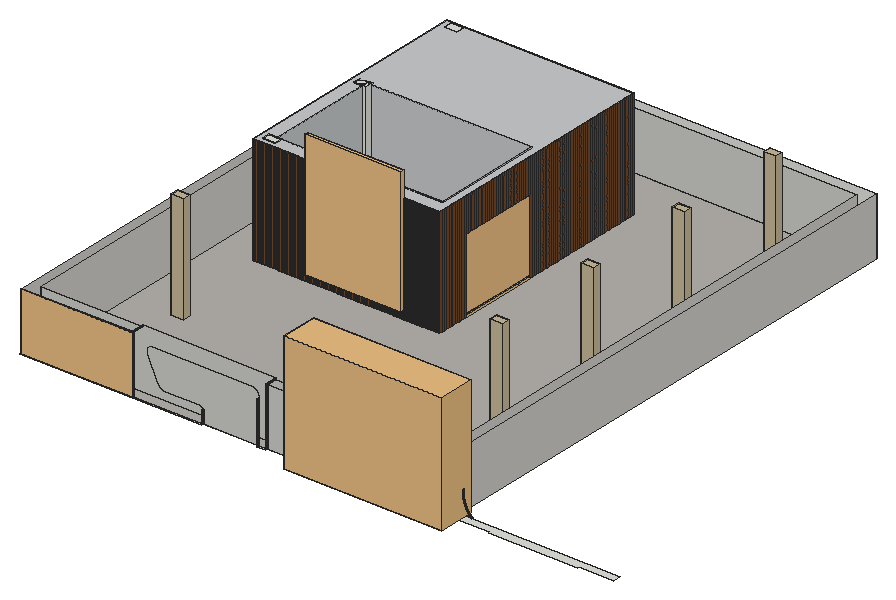
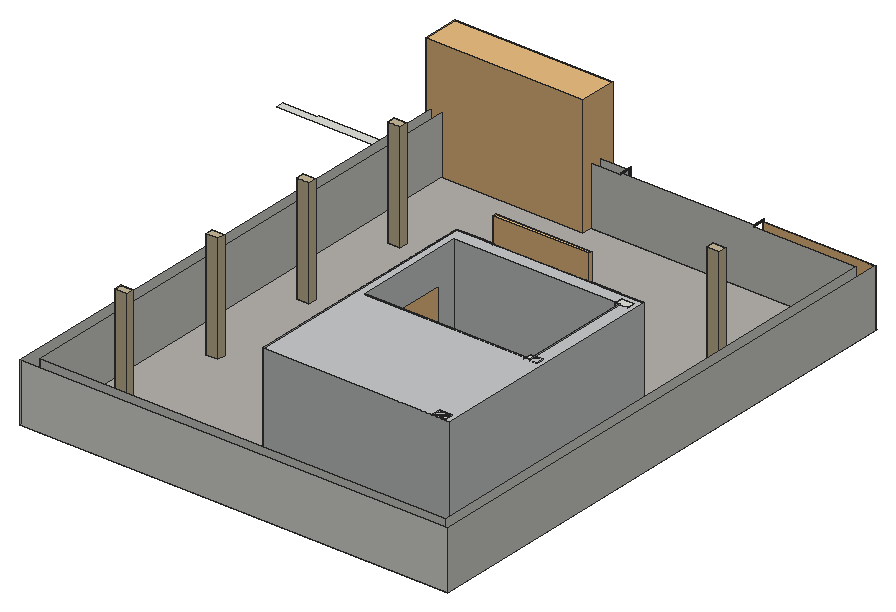
# SketchUp Ruby script. Lengths in inches.
U = 1.inch
M = Sketchup.active_model
def pt(a) = Geom::Point3d.new(a.map { |v| v * U })
def face(e, loops, mat)
  f = e.add_face(loops[0].map { |a| pt(a) })
  loops[1..].each { |l| e.add_face(l.map { |a| pt(a) }).erase! }
  f.material = f.back_material = mat if mat
  f
end
# faces: each face lists its corners as indices into pts; further lists are holes
def faces(e, pts, list, mat = nil) = list.each { |f| face(e, (f[0].is_a?(Array) ? f : [f]).map { |l| l.map { |i| pts[i] } }, mat) }
# xy, xz, yz: faces in a plane at the given z, y or x. An outline is a flat list of corners, or four numbers for a rectangle; further outlines are holes
def ring(l) = l.size == 4 ? [[l[0], l[1]], [l[2], l[1]], [l[2], l[3]], [l[0], l[3]]] : l.each_slice(2).to_a
def flat(e, list, mat, &to3) = list.each { |f| face(e, (f[0].is_a?(Array) ? f : [f]).map { |l| ring(l).map { |u, v| to3.(u, v) } }, mat) }
def xy(e, z, list, mat = nil) = flat(e, list, mat) { |x, y| [x, y, z] }
def xz(e, y, list, mat = nil) = flat(e, list, mat) { |x, z| [x, y, z] }
def yz(e, x, list, mat = nil) = flat(e, list, mat) { |y, z| [x, y, z] }
def lines(e, pts, list) = list.each { |a, b| e.add_line(pt(pts[a]), pt(pts[b])) }
# prism: a flat outline (further loops are holes) pulled along v
def prism(e, loops, v, mat = nil)
  f = face(e, loops, mat); d = Geom::Vector3d.new(v.map { |x| x * U })
  f.pushpull(f.normal.samedirection?(d) ? d.length : -d.length)
end
def box(e, o, s, mat = nil) = prism(e, [[o, [o[0] + s[0], o[1], o[2]], [o[0] + s[0], o[1] + s[1], o[2]], [o[0], o[1] + s[1], o[2]]]], [0, 0, s[2]], mat)
def at(x, y, z, deg = 0) = Geom::Transformation.translation(pt([x, y, z])) * Geom::Transformation.rotation(ORIGIN, Z_AXIS, deg.degrees)
def axes(o, x, y, z) = Geom::Transformation.new([*x, 0, *y, 0, *z, 0, *pt(o).to_a, 1])
def part(name) = M.definitions.add(name)
# library, detail: a bought-in or finely detailed component or shape, given as its bounding box
def library(name, o, s) = part(name).tap { |d| box(d.entities, o, s) }
def detail(e, o, s) = box(e.add_group.entities, o, s)
def put(e, d, t, mat = nil) = e.add_instance(d, t).tap { |i| i.material = mat if mat }
def group(e, t, mat = nil) = e.add_group.tap { |g| g.transformation = t; g.material = mat if mat }.entities
root = M.entities
M.materials.add("1443 AP 8258 WINTER MOON").color = [199, 202, 203]
M.materials.add("[Granite Dark Gray]").color = [51, 50, 50]
M.materials.add("[Quartz Light Brown]").color = [199, 184, 152]
M.materials.add("[Stone Sandstone Ashlar Light]").color = [206, 205, 201]
M.materials.add("[Tile Travertine 2 inch]").color = [181, 178, 172]
M.materials.add("[Wood Cherry Original]").color = [118, 74, 44]
c1 = library("Group\#32",[0,-1,0],[125.5,1,65])
c2 = library("cong+trinh+1",[39.36,9.05,6.78],[177.14,41.14,133.75])
c3 = part("5")
box(c3.entities,[0,0,0],[14,9,121.75])
c4 = library("Plant wall",[-73.82,-5.93,-13.13],[107,4.1,140.96])
c5 = part("Group519\#1")
box(c5.entities,[-105,-60.875,0],[2.5,121.75,0.5])
c6 = part("Group520\#1")
box(c6.entities,[-102,-60.875,0],[2.5,121.75,0.5])
c7 = part("Group521\#1")
box(c7.entities,[-99,-60.875,0],[2.5,121.75,0.5])
c8 = part("Group522\#1")
box(c8.entities,[-96,-60.875,0],[2.5,121.75,0.5])
c9 = part("Group523\#1")
box(c9.entities,[-93,-60.875,0],[2.5,121.75,0.5])
c10 = part("Group524\#1")
box(c10.entities,[-90,-60.875,0],[2.5,121.75,0.5])
c11 = part("Group525\#1")
box(c11.entities,[-87,-60.875,0],[2.5,121.75,0.5])
c12 = part("Group526\#1")
box(c12.entities,[-84,-60.875,0],[2.5,121.75,0.5])
c13 = part("Group527\#1")
box(c13.entities,[-81,-60.875,0],[2.5,121.75,0.5])
c14 = part("Group528\#1")
box(c14.entities,[-78,-60.875,0],[2.5,121.75,0.5])
c15 = part("Group529\#1")
box(c15.entities,[-75,-60.875,0],[2.5,121.75,0.5])
c16 = part("Group530\#1")
box(c16.entities,[-72,-60.875,0],[2.5,121.75,0.5])
c17 = part("Group531\#1")
box(c17.entities,[-69,-60.875,0],[2.5,121.75,0.5])
c18 = part("Group532\#1")
box(c18.entities,[-66,-60.875,0],[2.5,121.75,0.5])
c19 = part("Group533\#1")
box(c19.entities,[-63,-60.875,0],[2.5,121.75,0.5])
c20 = part("Group534\#1")
box(c20.entities,[-60,-60.875,0],[2.5,121.75,0.5])
c21 = part("Group535\#1")
box(c21.entities,[-57,-60.875,0],[2.5,121.75,0.5])
c22 = part("Group536\#1")
box(c22.entities,[-54,-60.875,0],[2.5,121.75,0.5])
c23 = part("Group537\#1")
box(c23.entities,[-51,-60.875,0],[2.5,121.75,0.5])
c24 = part("Group538\#1")
box(c24.entities,[-48,-60.875,0],[2.5,121.75,0.5])
c25 = part("Group539\#1")
box(c25.entities,[-45,-60.875,0],[2.5,121.75,0.5])
c26 = part("Group540\#1")
box(c26.entities,[-42,-60.875,0],[2.5,121.75,0.5])
c27 = part("Group541\#1")
xy(c27.entities,0,[[-39,-60.875,-36.5,-36.875]])
xy(c27.entities,0.5,[[-39,-60.875,-36.5,-36.875]])
xz(c27.entities,-60.875,[[-39,0,-36.5,0.5]])
yz(c27.entities,-39,[[-60.875,0,-36.875,0.5],[-36.875,0,60.875,0.5]])
yz(c27.entities,-36.5,[[-60.875,0,-36.875,0.5]])
c28 = part("Group542\#1")
box(c28.entities,[-36,-60.875,0],[2.5,24,0.5])
c29 = part("Group543\#1")
box(c29.entities,[-33,-60.875,0],[2.5,24,0.5])
c30 = part("Group544\#1")
box(c30.entities,[-30,-60.875,0],[2.5,24,0.5])
c31 = part("Group545\#1")
box(c31.entities,[-27,-60.875,0],[2.5,24,0.5])
c32 = part("Group546\#1")
box(c32.entities,[-24,-60.875,0],[2.5,24,0.5])
c33 = part("Group547\#1")
box(c33.entities,[-21,-60.875,0],[2.5,24,0.5])
c34 = part("Group548\#1")
box(c34.entities,[-18,-60.875,0],[2.5,24,0.5])
c35 = part("Group549\#1")
box(c35.entities,[-15,-60.875,0],[2.5,24,0.5])
c36 = part("Group550\#1")
box(c36.entities,[-12,-60.875,0],[2.5,24,0.5])
c37 = part("Group551\#1")
box(c37.entities,[-9,-60.875,0],[2.5,24,0.5])
c38 = part("Group552\#1")
box(c38.entities,[-6,-60.875,0],[2.5,24,0.5])
c39 = part("Group553\#1")
box(c39.entities,[-3,-60.875,0],[2.5,24,0.5])
c40 = part("Group554\#1")
box(c40.entities,[0,-60.875,0],[2.5,24,0.5])
c41 = part("Group555\#1")
box(c41.entities,[3,-60.875,0],[2.5,24,0.5])
c42 = part("Group556\#1")
box(c42.entities,[6,-60.875,0],[2.5,24,0.5])
c43 = part("Group557\#1")
box(c43.entities,[9,-60.875,0],[2.5,24,0.5])
c44 = part("Group558\#1")
box(c44.entities,[12,-60.875,0],[2.5,24,0.5])
c45 = part("Group559\#1")
box(c45.entities,[15,-60.875,0],[2.5,24,0.5])
c46 = part("Group560\#1")
box(c46.entities,[18,-60.875,0],[2.5,24,0.5])
c47 = part("Group561\#1")
box(c47.entities,[21,-60.875,0],[2.5,24,0.5])
c48 = part("Group562\#1")
box(c48.entities,[24,-60.875,0],[2.5,24,0.5])
c49 = part("Group563\#1")
box(c49.entities,[27,-60.875,0],[2.5,24,0.5])
c50 = part("Group564\#1")
box(c50.entities,[30,-60.875,0],[2.5,24,0.5])
c51 = part("Group565\#1")
box(c51.entities,[33,-60.875,0],[2.5,24,0.5])
c52 = part("Group566\#1")
box(c52.entities,[36,-60.875,0],[2.5,24,0.5])
c53 = part("Group567\#1")
box(c53.entities,[39,-60.875,0],[2.5,24,0.5])
c54 = part("Group568\#1")
box(c54.entities,[42,-60.875,0],[2.5,24,0.5])
c55 = part("Group569\#1")
box(c55.entities,[45,-60.875,0],[2.5,24,0.5])
c56 = part("Group570\#1")
box(c56.entities,[48,-60.875,0],[2.5,24,0.5])
c57 = part("Group571\#1")
box(c57.entities,[51,-60.875,0],[2.5,24,0.5])
c58 = part("Group572\#1")
box(c58.entities,[54,-60.875,0],[2.5,24,0.5])
c59 = part("Group573\#1")
prism(c59.entities,[[[57,-36.875,0],[57,60.875,0],[59.5,60.875,0],[59.5,-60.875,0],[57,-60.875,0]]],[0,0,0.5])
c60 = part("Group574\#1")
box(c60.entities,[60,-60.875,0],[2.5,121.75,0.5])
c61 = part("Group575\#1")
box(c61.entities,[63,-60.875,0],[2.5,121.75,0.5])
c62 = part("Group576\#1")
box(c62.entities,[66,-60.875,0],[2.5,121.75,0.5])
c63 = part("Group577\#1")
box(c63.entities,[69,-60.875,0],[2.5,121.75,0.5])
c64 = part("Group578\#1")
box(c64.entities,[72,-60.875,0],[2.5,121.75,0.5])
c65 = part("Group579\#1")
box(c65.entities,[75,-60.875,0],[2.5,121.75,0.5])
c66 = part("Group580\#1")
box(c66.entities,[78,-60.875,0],[2.5,121.75,0.5])
c67 = part("Group581\#1")
box(c67.entities,[81,-60.875,0],[2.5,121.75,0.5])
c68 = part("Group582\#1")
box(c68.entities,[84,-60.875,0],[2.5,121.75,0.5])
c69 = part("Group583\#1")
box(c69.entities,[87,-60.875,0],[2.5,121.75,0.5])
c70 = part("Group584\#1")
box(c70.entities,[90,-60.875,0],[2.5,121.75,0.5])
c71 = part("Group585\#1")
box(c71.entities,[93,-60.875,0],[2.5,121.75,0.5])
c72 = part("Group586\#1")
box(c72.entities,[96,-60.875,0],[2.5,121.75,0.5])
c73 = part("Group587\#1")
box(c73.entities,[99,-60.875,0],[2.5,121.75,0.5])
c74 = part("Group588\#1")
box(c74.entities,[102,-60.875,0],[2.5,121.75,0.5])
c75 = part("Group517\#1")
put(c75.entities,c5,at(0,0,0))
put(c75.entities,c6,at(0,0,0))
put(c75.entities,c7,at(0,0,0))
put(c75.entities,c8,at(0,0,0))
put(c75.entities,c9,at(0,0,0))
put(c75.entities,c10,at(0,0,0))
put(c75.entities,c11,at(0,0,0))
put(c75.entities,c12,at(0,0,0))
put(c75.entities,c13,at(0,0,0))
put(c75.entities,c14,at(0,0,0))
put(c75.entities,c15,at(0,0,0))
put(c75.entities,c16,at(0,0,0))
put(c75.entities,c17,at(0,0,0))
put(c75.entities,c18,at(0,0,0))
put(c75.entities,c19,at(0,0,0))
put(c75.entities,c20,at(0,0,0))
put(c75.entities,c21,at(0,0,0))
put(c75.entities,c22,at(0,0,0))
put(c75.entities,c23,at(0,0,0))
put(c75.entities,c24,at(0,0,0))
put(c75.entities,c25,at(0,0,0))
put(c75.entities,c26,at(0,0,0))
put(c75.entities,c27,at(0,0,0))
put(c75.entities,c28,at(0,0,0))
put(c75.entities,c29,at(0,0,0))
put(c75.entities,c30,at(0,0,0))
put(c75.entities,c31,at(0,0,0))
put(c75.entities,c32,at(0,0,0))
put(c75.entities,c33,at(0,0,0))
put(c75.entities,c34,at(0,0,0))
put(c75.entities,c35,at(0,0,0))
put(c75.entities,c36,at(0,0,0))
put(c75.entities,c37,at(0,0,0))
put(c75.entities,c38,at(0,0,0))
put(c75.entities,c39,at(0,0,0))
put(c75.entities,c40,at(0,0,0))
put(c75.entities,c41,at(0,0,0))
put(c75.entities,c42,at(0,0,0))
put(c75.entities,c43,at(0,0,0))
put(c75.entities,c44,at(0,0,0))
put(c75.entities,c45,at(0,0,0))
put(c75.entities,c46,at(0,0,0))
put(c75.entities,c47,at(0,0,0))
put(c75.entities,c48,at(0,0,0))
put(c75.entities,c49,at(0,0,0))
put(c75.entities,c50,at(0,0,0))
put(c75.entities,c51,at(0,0,0))
put(c75.entities,c52,at(0,0,0))
put(c75.entities,c53,at(0,0,0))
put(c75.entities,c54,at(0,0,0))
put(c75.entities,c55,at(0,0,0))
put(c75.entities,c56,at(0,0,0))
put(c75.entities,c57,at(0,0,0))
put(c75.entities,c58,at(0,0,0))
put(c75.entities,c59,at(0,0,0))
put(c75.entities,c60,at(0,0,0))
put(c75.entities,c61,at(0,0,0))
put(c75.entities,c62,at(0,0,0))
put(c75.entities,c63,at(0,0,0))
put(c75.entities,c64,at(0,0,0))
put(c75.entities,c65,at(0,0,0))
put(c75.entities,c66,at(0,0,0))
put(c75.entities,c67,at(0,0,0))
put(c75.entities,c68,at(0,0,0))
put(c75.entities,c69,at(0,0,0))
put(c75.entities,c70,at(0,0,0))
put(c75.entities,c71,at(0,0,0))
put(c75.entities,c72,at(0,0,0))
put(c75.entities,c73,at(0,0,0))
put(c75.entities,c74,at(0,0,0))
c76 = library("SLIDING+GLASS+DOOR\#1",[0,-0.75,0],[72,5.75,80])
c77 = part("Group591\#1")
box(c77.entities,[-136,-60.875,0],[2.5,121.75,0.5])
c78 = part("Group592\#1")
box(c78.entities,[-133,-60.875,0],[2.5,121.75,0.5])
c79 = part("Group593\#1")
box(c79.entities,[-130,-60.875,0],[2.5,121.75,0.5])
c80 = part("Group594\#1")
box(c80.entities,[-127,-60.875,0],[2.5,121.75,0.5])
c81 = part("Group595\#1")
box(c81.entities,[-124,-60.875,0],[2.5,121.75,0.5])
c82 = part("Group596\#1")
box(c82.entities,[-121,-60.875,0],[2.5,121.75,0.5])
c83 = part("Group597\#1")
box(c83.entities,[-118,-60.875,0],[2.5,121.75,0.5])
c84 = part("Group598\#1")
box(c84.entities,[-115,-60.875,0],[2.5,121.75,0.5])
c85 = part("Group599\#1")
box(c85.entities,[-112,-60.875,0],[2.5,121.75,0.5])
c86 = part("Group600\#1")
box(c86.entities,[-109,-60.875,0],[2.5,121.75,0.5])
c87 = part("Group601\#1")
box(c87.entities,[-106,-60.875,0],[2.5,121.75,0.5])
c88 = part("Group602\#1")
box(c88.entities,[-103,-60.875,0],[2.5,121.75,0.5])
c89 = part("Group604\#1")
box(c89.entities,[-97,23.125,0],[2.5,37.75,0.5])
c90 = part("Group605\#1")
box(c90.entities,[-94,23.125,0],[2.5,37.75,0.5])
c91 = part("Group606\#1")
box(c91.entities,[-91,23.125,0],[2.5,37.75,0.5])
c92 = part("Group607\#1")
box(c92.entities,[-88,23.125,0],[2.5,37.75,0.5])
c93 = part("Group608\#1")
box(c93.entities,[-85,23.125,0],[2.5,37.75,0.5])
c94 = part("Group609\#1")
box(c94.entities,[-82,23.125,0],[2.5,37.75,0.5])
c95 = part("Group610\#1")
box(c95.entities,[-79,23.125,0],[2.5,37.75,0.5])
c96 = part("Group611\#1")
box(c96.entities,[-76,23.125,0],[2.5,37.75,0.5])
c97 = part("Group612\#1")
box(c97.entities,[-73,23.125,0],[2.5,37.75,0.5])
c98 = part("Group613\#1")
box(c98.entities,[-70,23.125,0],[2.5,37.75,0.5])
c99 = part("Group614\#1")
box(c99.entities,[-67,23.125,0],[2.5,37.75,0.5])
c100 = part("Group615\#1")
box(c100.entities,[-64,23.125,0],[2.5,37.75,0.5])
c101 = part("Group616\#1")
box(c101.entities,[-61,23.125,0],[2.5,37.75,0.5])
c102 = part("Group617\#1")
box(c102.entities,[-58,23.125,0],[2.5,37.75,0.5])
c103 = part("Group618\#1")
box(c103.entities,[-55,23.125,0],[2.5,37.75,0.5])
c104 = part("Group619\#1")
box(c104.entities,[-52,23.125,0],[2.5,37.75,0.5])
c105 = part("Group620\#1")
box(c105.entities,[-49,23.125,0],[2.5,37.75,0.5])
c106 = part("Group621\#1")
box(c106.entities,[-46,23.125,0],[2.5,37.75,0.5])
c107 = part("Group622\#1")
box(c107.entities,[-43,23.125,0],[2.5,37.75,0.5])
c108 = part("Group623\#1")
box(c108.entities,[-40,23.125,0],[2.5,37.75,0.5])
c109 = part("Group624\#1")
box(c109.entities,[-37,23.125,0],[2.5,37.75,0.5])
c110 = part("Group625\#1")
box(c110.entities,[-34,23.125,0],[2.5,37.75,0.5])
c111 = part("Group626\#1")
box(c111.entities,[-31,23.125,0],[2.5,37.75,0.5])
c112 = part("Group627\#1")
box(c112.entities,[-28,23.125,0],[2.5,37.75,0.5])
c113 = part("Group628\#1")
box(c113.entities,[-25,23.125,0],[2.5,37.75,0.5])
c114 = part("Group629\#1")
box(c114.entities,[-22,23.125,0],[2.5,37.75,0.5])
c115 = part("Group630\#1")
box(c115.entities,[-19,23.125,0],[2.5,37.75,0.5])
c116 = part("Group631\#1")
box(c116.entities,[-16,23.125,0],[2.5,37.75,0.5])
c117 = part("Group632\#1")
box(c117.entities,[-13,23.125,0],[2.5,37.75,0.5])
c118 = part("Group633\#1")
prism(c118.entities,[[[-7.5,60.875,0],[-7.5,-60.875,0],[-10,-60.875,0],[-10,-58.875,0],[-10,23.125,0],[-10,60.875,0]]],[0,0,0.5])
c119 = part("Group634\#1")
box(c119.entities,[-7,-60.875,0],[2.5,121.75,0.5])
c120 = part("Group635\#1")
box(c120.entities,[-4,-60.875,0],[2.5,121.75,0.5])
c121 = part("Group636\#1")
box(c121.entities,[-1,-60.875,0],[2.5,121.75,0.5])
c122 = part("Group637\#1")
box(c122.entities,[2,-60.875,0],[2.5,121.75,0.5])
c123 = part("Group638\#1")
box(c123.entities,[5,-60.875,0],[2.5,121.75,0.5])
c124 = part("Group639\#1")
box(c124.entities,[8,-60.875,0],[2.5,121.75,0.5])
c125 = part("Group640\#1")
box(c125.entities,[11,-60.875,0],[2.5,121.75,0.5])
c126 = part("Group641\#1")
box(c126.entities,[14,-60.875,0],[2.5,121.75,0.5])
c127 = part("Group642\#1")
box(c127.entities,[17,-60.875,0],[2.5,121.75,0.5])
c128 = part("Group643\#1")
box(c128.entities,[20,-60.875,0],[2.5,121.75,0.5])
c129 = part("Group644\#1")
box(c129.entities,[23,-60.875,0],[2.5,121.75,0.5])
c130 = part("Group645\#1")
box(c130.entities,[26,-60.875,0],[2.5,121.75,0.5])
c131 = part("Group646\#1")
box(c131.entities,[29,-60.875,0],[2.5,121.75,0.5])
c132 = part("Group647\#1")
box(c132.entities,[32,-60.875,0],[2.5,121.75,0.5])
c133 = part("Group648\#1")
box(c133.entities,[35,-60.875,0],[2.5,121.75,0.5])
c134 = part("Group649\#1")
box(c134.entities,[38,-60.875,0],[2.5,121.75,0.5])
c135 = part("Group650\#1")
box(c135.entities,[41,-60.875,0],[2.5,121.75,0.5])
c136 = part("Group651\#1")
box(c136.entities,[44,-60.875,0],[2.5,121.75,0.5])
c137 = part("Group652\#1")
box(c137.entities,[47,-60.875,0],[2.5,121.75,0.5])
c138 = part("Group653\#1")
box(c138.entities,[50,-60.875,0],[2.5,121.75,0.5])
c139 = part("Group654\#1")
box(c139.entities,[53,-60.875,0],[2.5,121.75,0.5])
c140 = part("Group655\#1")
box(c140.entities,[56,-60.875,0],[2.5,121.75,0.5])
c141 = part("Group656\#1")
box(c141.entities,[59,-60.875,0],[2.5,121.75,0.5])
c142 = part("Group657\#1")
box(c142.entities,[62,-60.875,0],[2.5,121.75,0.5])
c143 = part("Group658\#1")
box(c143.entities,[65,-60.875,0],[2.5,121.75,0.5])
c144 = part("Group659\#1")
box(c144.entities,[68,-60.875,0],[2.5,121.75,0.5])
c145 = part("Group660\#1")
box(c145.entities,[71,-60.875,0],[2.5,121.75,0.5])
c146 = part("Group661\#1")
box(c146.entities,[74,-60.875,0],[2.5,121.75,0.5])
c147 = part("Group662\#1")
box(c147.entities,[77,-60.875,0],[2.5,121.75,0.5])
c148 = part("Group663\#1")
box(c148.entities,[80,-60.875,0],[2.5,121.75,0.5])
c149 = part("Group664\#1")
box(c149.entities,[83,-60.875,0],[2.5,121.75,0.5])
c150 = part("Group665\#1")
box(c150.entities,[86,-60.875,0],[2.5,121.75,0.5])
c151 = part("Group666\#1")
box(c151.entities,[89,-60.875,0],[2.5,121.75,0.5])
c152 = part("Group667\#1")
box(c152.entities,[92,-60.875,0],[2.5,121.75,0.5])
c153 = part("Group668\#1")
box(c153.entities,[95,-60.875,0],[2.5,121.75,0.5])
c154 = part("Group669\#1")
box(c154.entities,[98,-60.875,0],[2.5,121.75,0.5])
c155 = part("Group670\#1")
box(c155.entities,[101,-60.875,0],[2.5,121.75,0.5])
c156 = part("Group671\#1")
box(c156.entities,[104,-60.875,0],[2.5,121.75,0.5])
c157 = part("Group672\#1")
box(c157.entities,[107,-60.875,0],[2.5,121.75,0.5])
c158 = part("Group673\#1")
box(c158.entities,[110,-60.875,0],[2.5,121.75,0.5])
c159 = part("Group674\#1")
box(c159.entities,[113,-60.875,0],[2.5,121.75,0.5])
c160 = part("Group675\#1")
box(c160.entities,[116,-60.875,0],[2.5,121.75,0.5])
c161 = part("Group676\#1")
box(c161.entities,[119,-60.875,0],[2.5,121.75,0.5])
c162 = part("Group677\#1")
box(c162.entities,[122,-60.875,0],[2.5,121.75,0.5])
c163 = part("Group678\#1")
box(c163.entities,[125,-60.875,0],[2.5,121.75,0.5])
c164 = part("Group679\#1")
box(c164.entities,[128,-60.875,0],[2.5,121.75,0.5])
c165 = part("Group680\#1")
box(c165.entities,[131,-60.875,0],[2.5,121.75,0.5])
c166 = part("Group681\#1")
xy(c166.entities,0,[[134,-60.875,136,60.875]])
xy(c166.entities,0.5,[[134,-60.875,136,60.875]])
yz(c166.entities,134,[[-60.875,0,60.875,0.5]])
c167 = part("Group589\#1")
put(c167.entities,c77,at(0,0,0))
put(c167.entities,c78,at(0,0,0))
put(c167.entities,c79,at(0,0,0))
put(c167.entities,c80,at(0,0,0))
put(c167.entities,c81,at(0,0,0))
put(c167.entities,c82,at(0,0,0))
put(c167.entities,c83,at(0,0,0))
put(c167.entities,c84,at(0,0,0))
put(c167.entities,c85,at(0,0,0))
put(c167.entities,c86,at(0,0,0))
put(c167.entities,c87,at(0,0,0))
put(c167.entities,c88,at(0,0,0))
put(c167.entities,c89,at(0,0,0))
put(c167.entities,c90,at(0,0,0))
put(c167.entities,c91,at(0,0,0))
put(c167.entities,c92,at(0,0,0))
put(c167.entities,c93,at(0,0,0))
put(c167.entities,c94,at(0,0,0))
put(c167.entities,c95,at(0,0,0))
put(c167.entities,c96,at(0,0,0))
put(c167.entities,c97,at(0,0,0))
put(c167.entities,c98,at(0,0,0))
put(c167.entities,c99,at(0,0,0))
put(c167.entities,c100,at(0,0,0))
put(c167.entities,c101,at(0,0,0))
put(c167.entities,c102,at(0,0,0))
put(c167.entities,c103,at(0,0,0))
put(c167.entities,c104,at(0,0,0))
put(c167.entities,c105,at(0,0,0))
put(c167.entities,c106,at(0,0,0))
put(c167.entities,c107,at(0,0,0))
put(c167.entities,c108,at(0,0,0))
put(c167.entities,c109,at(0,0,0))
put(c167.entities,c110,at(0,0,0))
put(c167.entities,c111,at(0,0,0))
put(c167.entities,c112,at(0,0,0))
put(c167.entities,c113,at(0,0,0))
put(c167.entities,c114,at(0,0,0))
put(c167.entities,c115,at(0,0,0))
put(c167.entities,c116,at(0,0,0))
put(c167.entities,c117,at(0,0,0))
put(c167.entities,c118,at(0,0,0))
put(c167.entities,c119,at(0,0,0))
put(c167.entities,c120,at(0,0,0))
put(c167.entities,c121,at(0,0,0))
put(c167.entities,c122,at(0,0,0))
put(c167.entities,c123,at(0,0,0))
put(c167.entities,c124,at(0,0,0))
put(c167.entities,c125,at(0,0,0))
put(c167.entities,c126,at(0,0,0))
put(c167.entities,c127,at(0,0,0))
put(c167.entities,c128,at(0,0,0))
put(c167.entities,c129,at(0,0,0))
put(c167.entities,c130,at(0,0,0))
put(c167.entities,c131,at(0,0,0))
put(c167.entities,c132,at(0,0,0))
put(c167.entities,c133,at(0,0,0))
put(c167.entities,c134,at(0,0,0))
put(c167.entities,c135,at(0,0,0))
put(c167.entities,c136,at(0,0,0))
put(c167.entities,c137,at(0,0,0))
put(c167.entities,c138,at(0,0,0))
put(c167.entities,c139,at(0,0,0))
put(c167.entities,c140,at(0,0,0))
put(c167.entities,c141,at(0,0,0))
put(c167.entities,c142,at(0,0,0))
put(c167.entities,c143,at(0,0,0))
put(c167.entities,c144,at(0,0,0))
put(c167.entities,c145,at(0,0,0))
put(c167.entities,c146,at(0,0,0))
put(c167.entities,c147,at(0,0,0))
put(c167.entities,c148,at(0,0,0))
put(c167.entities,c149,at(0,0,0))
put(c167.entities,c150,at(0,0,0))
put(c167.entities,c151,at(0,0,0))
put(c167.entities,c152,at(0,0,0))
put(c167.entities,c153,at(0,0,0))
put(c167.entities,c154,at(0,0,0))
put(c167.entities,c155,at(0,0,0))
put(c167.entities,c156,at(0,0,0))
put(c167.entities,c157,at(0,0,0))
put(c167.entities,c158,at(0,0,0))
put(c167.entities,c159,at(0,0,0))
put(c167.entities,c160,at(0,0,0))
put(c167.entities,c161,at(0,0,0))
put(c167.entities,c162,at(0,0,0))
put(c167.entities,c163,at(0,0,0))
put(c167.entities,c164,at(0,0,0))
put(c167.entities,c165,at(0,0,0))
put(c167.entities,c166,at(0,0,0))
put(c167.entities,c89,at(-3,0,0))
c168 = library("Group680\#2",[-45,-1,0],[89.5,2,0.5])
xy(root,6,[[126,46,126,48,0,48,0,648,480,648,480,63,660,63,660,54,621,54,621,53,521,53,521,54,480,54,480,48,468,48,468,636,12,636,12,60,348,60,348,48,276,48,276,46,266,46,266,48,204,48,204,46]])
xy(root,6,[[[54,305,264,577],[69,320,255,446]]],"1443 AP 8258 WINTER MOON")
xy(root,6,[[0,46,126,46,126,48,468,48,468,63,480,63,480,648,0,648]],"[Tile Travertine 2 inch]")
xy(root,8,[[255,341,264,431]],"1443 AP 8258 WINTER MOON")
xy(root,21,[[309,48,339,55]],"[Stone Sandstone Ashlar Light]")
xy(root,90,[[255,341,264,431]],"1443 AP 8258 WINTER MOON")
xy(root,127.75,[[[54,305,264,577],[69,320,255,446]]],"1443 AP 8258 WINTER MOON")
xz(root,48,[[0,6,126,71],[204,6,266,6,266,54.16,265.99,54.3125,265.99,54.47,265.98,54.63,265.97,54.78,265.93,55.1,265.91,55.25,265.89,55.41,265.86,55.5625,265.83,55.72,265.77,56.02,265.73,56.18,265.61,56.63,265.46,57.08,265.4,57.23,265.34,57.37,265.28,57.52,265.16,57.8,265.09,57.95,264.95,58.23,264.87,58.36,264.71,58.64,264.55,58.9,264.28,59.29,264.1875,59.42,264.09,59.54,263.99,59.66,263.89,59.79,263.79,59.9,263.6875,60.02,263.58,60.14,263.14,60.58,263.02,60.6875,262.9,60.79,262.79,60.89,262.66,60.99,262.54,61.09,262.42,61.1875,262.29,61.28,261.9,61.55,261.64,61.71,261.36,61.87,261.23,61.95,260.95,62.09,260.8,62.16,260.52,62.28,260.37,62.34,260.23,62.4,260.08,62.46,259.63,62.61,259.18,62.73,259.02,62.77,258.72,62.83,258.5625,62.86,258.41,62.89,258.25,62.91,258.1,62.93,257.78,62.97,257.63,62.98,257.47,62.99,257.3125,62.99,257.16,63,146,63,145.87,62.98,145.74,62.95,145.61,62.93,145.48,62.9,145.36,62.86,145.23,62.83,145.1,62.79,144.98,62.75,144.86,62.7,144.73,62.65,144.49,62.55,144.37,62.49,144.25,62.4375,144.14,62.375,144.02,62.31,143.8,62.17,143.6875,62.1,143.58,62.03,143.47,61.95,143.37,61.87,143.26,61.79,143.16,61.7,143.06,61.62,142.97,61.53,142.87,61.4375,142.78,61.34,142.6875,61.25,142.6,61.15,142.51,61.05,142.35,60.85,142.27,60.74,142.19,60.64,142.05,60.42,141.98,60.3,141.91,60.19,141.85,60.08,141.67,59.72,141.52,59.36,141.48,59.23,141.4375,59.11,141.4,58.98,141.36,58.86,141.27,58.47,141.21,58.08,141.2,57.95,141.1875,57.82,141.18,57.6875,141.17,57.56,141.17,57.16,141.2,56.77,141.28,56.25,141.3125,56.12,141.34,55.99,141.375,55.86,141.41,55.74,141.45,55.61,141.49,55.49,141.54,55.36,141.69,55,153.23,30,153.31,29.83,153.39,29.67,153.48,29.5,153.57,29.34,153.66,29.17,153.75,29.01,153.85,28.86,154.05,28.54,154.27,28.24,154.375,28.09,154.49,27.94,154.61,27.8,154.72,27.65,154.85,27.51,154.97,27.375,155.1,27.24,155.22,27.1,155.36,26.97,155.49,26.84,155.625,26.72,155.76,26.59,155.9,26.47,156.05,26.35,156.19,26.23,156.34,26.12,156.48,26.01,156.64,25.9,156.79,25.79,156.94,25.6875,157.1,25.59,157.42,25.39,157.74,25.21,157.91,25.125,158.07,25.04,158.41,24.88,158.92,24.67,159.1,24.6,159.27,24.54,159.45,24.48,159.625,24.43,159.8,24.375,159.98,24.33,160.16,24.28,160.35,24.24,160.71,24.16,160.89,24.13,161.08,24.1,161.26,24.07,161.44,24.05,161.63,24.03,161.81,24.01,162,24,200.1,24,200.21,23.99,200.3125,23.99,200.42,23.98,200.52,23.97,200.73,23.93,200.93,23.89,201.04,23.86,201.14,23.84,201.24,23.8,201.34,23.77,201.43,23.73,201.53,23.7,201.625,23.65,201.72,23.61,201.82,23.5625,201.91,23.52,202,23.46,202.09,23.41,202.18,23.35,202.27,23.3,202.35,23.24,202.44,23.17,202.52,23.11,202.68,22.97,202.75,22.9,202.83,22.83,202.9,22.75,202.97,22.68,203.11,22.52,203.17,22.44,203.24,22.35,203.3,22.27,203.35,22.18,203.41,22.09,203.46,22,203.52,21.91,203.5625,21.82,203.61,21.72,203.65,21.625,203.7,21.53,203.73,21.43,203.77,21.34,203.8,21.24,203.84,21.14,203.86,21.04,203.89,20.93,203.93,20.73,203.97,20.52,203.98,20.42,203.99,20.3125,203.99,20.21,204,20.1],[[276,6,348,71],[309,21,339,57]],[468,6,480,71]],"[Stone Sandstone Ashlar Light]")
xz(root,55,[[309,21,339,57]],"[Granite Dark Gray]")
xz(root,60,[[12,6,12,71,126,71,126,73,276,73,276,71,348,71,348,6]],"[Stone Sandstone Ashlar Light]")
xz(root,305,[[54,6,264,6,264,127.75,216,127.75,216,30,120,30,120,127.75,54,127.75],[120,30,216,127.75]],"1443 AP 8258 WINTER MOON")
xz(root,320,[[69,6,255,127.75]],"1443 AP 8258 WINTER MOON")
xz(root,341,[[255,8,264,90]],"1443 AP 8258 WINTER MOON")
xz(root,431,[[255,8,264,90]],"1443 AP 8258 WINTER MOON")
xz(root,446,[[69,6,255,127.75]],"1443 AP 8258 WINTER MOON")
xz(root,577,[[54,6,264,127.75]],"1443 AP 8258 WINTER MOON")
xz(root,636,[[12,6,468,71]],"[Stone Sandstone Ashlar Light]")
xz(root,648,[[0,6,480,71]])
yz(root,0,[[48,6,648,71]],"[Stone Sandstone Ashlar Light]")
yz(root,12,[[60,6,636,71]],"[Stone Sandstone Ashlar Light]")
yz(root,54,[[305,6,577,127.75]],"1443 AP 8258 WINTER MOON")
yz(root,69,[[320,6,446,127.75]],"1443 AP 8258 WINTER MOON")
yz(root,126,[[46,6,46,73,60,73,60,71,48,71,48,6]],"[Granite Dark Gray]")
yz(root,203.99,[[46,20.21,48,20.3125]],"[Granite Dark Gray]")
yz(root,204,[[46,6,48,20],[46,20,48,20.1]],"[Granite Dark Gray]")
yz(root,255,[[[320,6,446,127.75],[341,8,431,90]]],"1443 AP 8258 WINTER MOON")
yz(root,264,[[[305,6,577,127.75],[341,8,431,90]]],"1443 AP 8258 WINTER MOON")
yz(root,266,[[46,6,48,54]],"[Granite Dark Gray]")
yz(root,276,[[46,6,48,6,48,71,60,71,60,73,46,73]],"[Granite Dark Gray]")
yz(root,309,[[48,21,55,57]],"[Stone Sandstone Ashlar Light]")
yz(root,339,[[48,21,55,57]],"[Stone Sandstone Ashlar Light]")
yz(root,348,[[48,6,60,71]],"[Stone Sandstone Ashlar Light]")
yz(root,468,[[48,6,636,71]],"[Stone Sandstone Ashlar Light]")
yz(root,480,[[48,6,54,6,54,65,63,65,63,6,648,6,648,71,48,71]],"[Stone Sandstone Ashlar Light]")
yz(root,491.5,[[53,35.04,54,35.5],[53,35.5,54,35.96]],"[Granite Dark Gray]")
p = [[501.15,54,13.68],[501.49,54,13.37],[501.49,53,13.37],[501.15,53,13.68],[500.81,54,14],[500.81,53,14],
  [500.47,54,14.32],[500.47,53,14.32],[500.14,54,14.64],[500.14,53,14.64],[499.82,54,14.97],[499.82,53,14.97],
  [499.5,54,15.31],[499.5,53,15.31],[499.18,54,15.65],[499.18,53,15.65],[498.87,54,15.99],[498.87,53,15.99],
  [498.57,54,16.34],[498.57,53,16.34],[498.27,54,16.7],[498.27,53,16.7],[497.98,54,17.06],[497.98,53,17.06],
  [497.69,54,17.42],[497.69,53,17.42],[497.41,54,17.79],[497.41,53,17.79],[497.13,54,18.16],[497.13,53,18.16],
  [496.86,54,18.54],[496.86,53,18.54],[496.6,54,18.92],[496.6,53,18.92],[496.34,54,19.3],[496.34,53,19.3],
  [496.09,54,19.69],[496.09,53,19.69],[495.85,54,20.09],[495.85,53,20.09],[203.99,46,20.21],[204,46,20.1],
  [204,48,20.1],[203.99,48,20.21],[495.61,54,20.48],[495.61,53,20.48],[203.98,46,20.42],[203.99,46,20.3125],
  [203.99,48,20.3125],[203.98,48,20.42],[203.97,46,20.52],[203.97,48,20.52],[203.95,46,20.625],[203.95,48,20.625],
  [495.375,54,20.88],[495.375,53,20.88],[203.93,46,20.73],[203.93,48,20.73],[203.91,46,20.83],[203.91,48,20.83],
  [203.89,46,20.93],[203.89,48,20.93],[203.86,46,21.04],[203.86,48,21.04],[495.15,54,21.29],[495.15,53,21.29],
  [203.84,46,21.14],[203.84,48,21.14],[203.8,46,21.24],[203.8,48,21.24],[203.77,46,21.34],[203.77,48,21.34],
  [203.73,46,21.43],[203.73,48,21.43],[494.93,54,21.7],[494.93,53,21.7],[494.72,54,22.11],[494.72,53,22.11],
  [494.51,54,22.52],[494.51,53,22.52],[494.31,54,22.94],[494.31,53,22.94],[494.11,54,23.36],[494.11,53,23.36],
  [493.93,54,23.78],[493.93,53,23.78],[493.75,54,24.21],[493.75,53,24.21],[493.57,54,24.64],[493.57,53,24.64],
  [493.4,54,25.07],[493.4,53,25.07],[493.24,54,25.51],[493.24,53,25.51],[493.09,54,25.94],[493.09,53,25.94],
  [492.94,54,26.38],[492.94,53,26.38],[492.8,54,26.83],[492.8,53,26.83],[492.67,54,27.27],[492.67,53,27.27],
  [492.55,54,27.72],[492.55,53,27.72],[492.43,54,28.16],[492.43,53,28.16],[492.32,54,28.61],[492.32,53,28.61],
  [492.21,54,29.06],[492.21,53,29.06],[492.11,54,29.52],[492.11,53,29.52],[492.02,54,29.97],[492.02,53,29.97],
  [491.9375,54,30.43],[491.9375,53,30.43],[491.86,54,30.89],[491.86,53,30.89],[491.79,54,31.34],[491.79,53,31.34],
  [491.73,54,31.8],[491.73,53,31.8],[491.68,54,32.26],[491.68,53,32.26],[491.63,54,32.72],[491.63,53,32.72],
  [491.59,54,33.19],[491.59,53,33.19],[491.56,54,33.65],[491.56,53,33.65],[491.53,54,34.11],[491.53,53,34.11],
  [491.51,54,34.57],[491.51,53,34.57],[491.5,54,35.04],[491.5,53,35.04],[491.51,54,36.43],[491.5,54,35.96],
  [491.5,53,35.96],[491.51,53,36.43],[491.53,54,36.89],[491.53,53,36.89],[491.56,54,37.35],[491.56,53,37.35],
  [491.59,54,37.81],[491.59,53,37.81],[491.63,54,38.28],[491.63,53,38.28],[491.68,54,38.74],[491.68,53,38.74],
  [491.73,54,39.2],[491.73,53,39.2],[156,48,24],[162,48,24],[153.23,48,30]]
faces(root,p,[[0,1,2,3],[4,0,3,5],[6,4,5,7],[8,6,7,9],[10,8,9,11],[12,10,11,13],[14,12,13,15],[16,14,15,17],
  [18,16,17,19],[20,18,19,21],[22,20,21,23],[24,22,23,25],[26,24,25,27],[28,26,27,29],[30,28,29,31],[32,30,31,33],
  [34,32,33,35],[36,34,35,37],[38,36,37,39],[40,41,42,43],[44,38,39,45],[46,47,48,49],[50,46,49,51],[52,50,51,53],
  [54,44,45,55],[56,52,53,57],[58,56,57,59],[60,58,59,61],[62,60,61,63],[64,54,55,65],[66,62,63,67],[68,66,67,69],
  [70,68,69,71],[72,70,71,73],[74,64,65,75],[76,74,75,77],[78,76,77,79],[80,78,79,81],[82,80,81,83],[84,82,83,85],
  [86,84,85,87],[88,86,87,89],[90,88,89,91],[92,90,91,93],[94,92,93,95],[96,94,95,97],[98,96,97,99],[100,98,99,101],
  [102,100,101,103],[104,102,103,105],[106,104,105,107],[108,106,107,109],[110,108,109,111],[112,110,111,113],[114,112,113,115],[116,114,115,117],
  [118,116,117,119],[120,118,119,121],[122,120,121,123],[124,122,123,125],[126,124,125,127],[128,126,127,129],[130,128,129,131],[132,130,131,133],
  [134,132,133,135],[136,137,138,139],[140,136,139,141],[142,140,141,143],[144,142,143,145],[146,144,145,147],[148,146,147,149],[150,148,149,151]],"[Granite Dark Gray]")
lines(root,p,[[152,153],[154,152]])
put(root,c1,at(0,48,6),"[Wood Cherry Original]")
put(root,c2,at(269.73,21.13,-0.78))
put(root,c3,at(60,183,6),"[Quartz Light Brown]")
put(root,c3,at(418,183,6),"[Quartz Light Brown]")
put(root,c4,at(190.04,306.83,28.01))
g1 = group(root,at(54,305,6),"[Wood Cherry Original]")
put(g1,c75,axes([105,0,60.875],[1,0,0],[0,0,1],[0,-1,0]))
put(root,c3,at(60,311,6))
put(root,c3,at(418,311,6),"[Quartz Light Brown]")
put(root,c76,axes([257.75,431,8],[-0.007,-1.25998,0],[0.99998,-0.00556,0],[0,0,1.025]))
g2 = group(root,at(264,305,6),"[Wood Cherry Original]")
put(g2,c167,axes([0,136,60.875],[0,1,0],[0,0,1],[1,0,0]))
put(g2,c168,axes([0,81,1],[0,1,0],[0,0,1],[1,0,0]))
put(root,c3,at(60,439,6))
put(root,c3,at(418,439,6),"[Quartz Light Brown]")
put(root,c3,at(60,567,6))
put(root,c3,at(418,567,6),"[Quartz Light Brown]")
